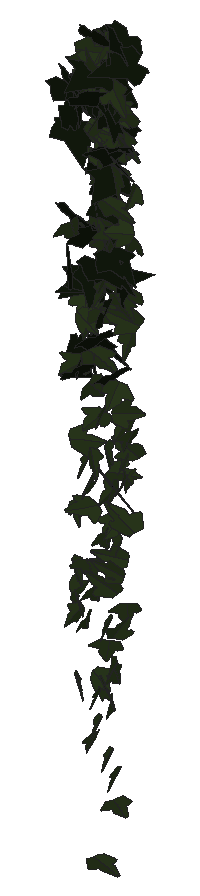
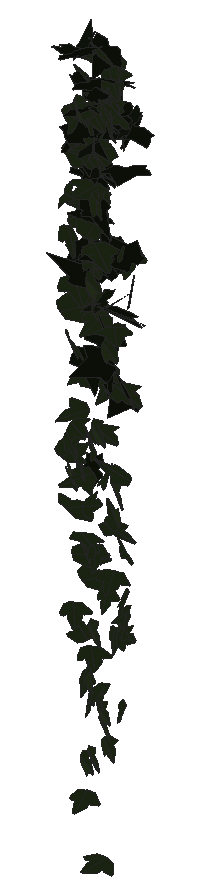
# SketchUp Ruby script. Lengths in inches.
U = 1.inch
M = Sketchup.active_model
def pt(a) = Geom::Point3d.new(a.map { |v| v * U })
def face(e, loops, mat)
  f = e.add_face(loops[0].map { |a| pt(a) })
  loops[1..].each { |l| e.add_face(l.map { |a| pt(a) }).erase! }
  f.material = f.back_material = mat if mat
  f
end
# faces: each face lists its corners as indices into pts; further lists are holes
def faces(e, pts, list, mat = nil) = list.each { |f| face(e, (f[0].is_a?(Array) ? f : [f]).map { |l| l.map { |i| pts[i] } }, mat) }
# xy, xz, yz: faces in a plane at the given z, y or x. An outline is a flat list of corners, or four numbers for a rectangle; further outlines are holes
def ring(l) = l.size == 4 ? [[l[0], l[1]], [l[2], l[1]], [l[2], l[3]], [l[0], l[3]]] : l.each_slice(2).to_a
def flat(e, list, mat, &to3) = list.each { |f| face(e, (f[0].is_a?(Array) ? f : [f]).map { |l| ring(l).map { |u, v| to3.(u, v) } }, mat) }
def xy(e, z, list, mat = nil) = flat(e, list, mat) { |x, y| [x, y, z] }
def xz(e, y, list, mat = nil) = flat(e, list, mat) { |x, z| [x, y, z] }
def yz(e, x, list, mat = nil) = flat(e, list, mat) { |y, z| [x, y, z] }
def lines(e, pts, list) = list.each { |a, b| e.add_line(pt(pts[a]), pt(pts[b])) }
# prism: a flat outline (further loops are holes) pulled along v
def prism(e, loops, v, mat = nil)
  f = face(e, loops, mat); d = Geom::Vector3d.new(v.map { |x| x * U })
  f.pushpull(f.normal.samedirection?(d) ? d.length : -d.length)
end
def box(e, o, s, mat = nil) = prism(e, [[o, [o[0] + s[0], o[1], o[2]], [o[0] + s[0], o[1] + s[1], o[2]], [o[0], o[1] + s[1], o[2]]]], [0, 0, s[2]], mat)
def at(x, y, z, deg = 0) = Geom::Transformation.translation(pt([x, y, z])) * Geom::Transformation.rotation(ORIGIN, Z_AXIS, deg.degrees)
def axes(o, x, y, z) = Geom::Transformation.new([*x, 0, *y, 0, *z, 0, *pt(o).to_a, 1])
def part(name) = M.definitions.add(name)
# library, detail: a bought-in or finely detailed component or shape, given as its bounding box
def library(name, o, s) = part(name).tap { |d| box(d.entities, o, s) }
def detail(e, o, s) = box(e.add_group.entities, o, s)
def put(e, d, t, mat = nil) = e.add_instance(d, t).tap { |i| i.material = mat if mat }
def group(e, t, mat = nil) = e.add_group.tap { |g| g.transformation = t; g.material = mat if mat }.entities
root = M.entities
M.materials.add("1026 AP 7946 SUNNY SIDE UP").color = [254, 231, 186]
M.materials.add("efeu1").color = [18, 25, 13]
M.materials.add("efeu2").color = [43, 57, 29]
c1 = part("ivyleaf_10")
p = [[0,0.5,-0.03],[-0.0625,2.02,-0.43],[-0.19,2.01,-0.46],[-0.54,1.05,-0.29],[-0.52,0.625,-0.18],[-0.83,0.76,-0.28],
  [-1.16,0.64,-0.33],[-1.15,0.33,-0.24],[-0.77,-0.39,0.02],[-0.3,-0.51,0.16],[0.04,-0.48,0.23],[-0.02,2.01,-0.4375],
  [-0.06,2.01,-0.43],[0.04,-0.49,0.23],[0.67,-0.49,0.14],[1.38,0.36,-0.2],[1.375,0.51,-0.24],[0.81,0.65,-0.19],
  [0.62,0.59,-0.15],[0.6,1.09,-0.28],[0.5,1.23,-0.31]]
faces(c1.entities,p,[[0,1,2,3,4,5,6,7,8,9,10],[11,12,0,13,14,15,16,17,18,19,20]],"efeu2")
c2 = part("ivyleaf_9")
p = [[1.54,2.16,1.25],[1.36,2.04,1.19],[-0.21,0.99,0.68],[-0.71,1.11,0.82],[-0.85,0.86,0.67],[-0.8,0.17,0.21],
  [-0.9,-0.01,0.1],[-0.67,-0.16,-0.02],[-0.08,-0.08,-0.05],[-0.03,-0.6,-0.4],[0.65,-0.88,-0.66],[0.83,-0.6,-0.49],
  [1.29,-0.42,-0.43],[1.8125,-0.07,-0.26],[1.21,0.44,0.15]]
faces(c2.entities,p,[[0,1,2,3,4,5,6,7,8,9,10,11,12,13,14]],"efeu1")
put(root,c1,axes([98.62,212.23,263.32],[-0.05399,0.08645,0.22814],[-0.03288,-0.21426,0.08745],[0.38721,-0.00614,0.03923]),"1026 AP 7946 SUNNY SIDE UP")
put(root,c2,axes([98,211.99,260.79],[0.05142,0.24508,-0.03116],[-0.00161,-0.03243,-0.26481],[-0.41963,0.03016,-0.0028]),"1026 AP 7946 SUNNY SIDE UP")
put(root,c1,axes([98.45,212.15,259.72],[0.16879,0.18196,-0.11803],[-0.09954,-0.09627,-0.22328],[-0.34936,0.11534,0.00659]),"1026 AP 7946 SUNNY SIDE UP")
put(root,c2,axes([98.13,212.12,257.58],[0.3163,-0.15076,0.02596],[0.01253,-0.03266,-0.25823],[0.24024,0.20019,-0.02071]),"1026 AP 7946 SUNNY SIDE UP")
put(root,c2,axes([97.9,212.27,266.85],[-0.38265,-0.11485,0.06292],[-0.02358,-0.09878,-0.25851],[0.21891,-0.21139,0.08214]),"1026 AP 7946 SUNNY SIDE UP")
put(root,c1,axes([98.48,212.1,255.43],[-0.08172,0.01136,-0.21221],[-0.32167,0.0251,0.05473],[0.04267,0.21102,0.00617]),"1026 AP 7946 SUNNY SIDE UP")
put(root,c2,axes([97.66,211.95,266.27],[0.24436,0.15063,0.08953],[0.11877,0.04568,-0.22161],[-0.2655,0.15907,-0.01674]),"1026 AP 7946 SUNNY SIDE UP")
put(root,c1,axes([98.14,212.25,258.12],[-0.02963,-0.00183,-0.24696],[0.14153,-0.22291,-0.00684],[-0.34936,-0.09015,0.01818]),"1026 AP 7946 SUNNY SIDE UP")
put(root,c1,axes([98.31,212.14,254.99],[-0.19456,-0.027,-0.19945],[-0.3045,-0.01293,0.12939],[-0.04009,0.22927,-0.01483]),"1026 AP 7946 SUNNY SIDE UP")
put(root,c2,axes([97.34,212.02,261.84],[-0.01147,-0.1083,0.21727],[0.07431,0.20015,0.1179],[-0.38551,0.0418,0.01626]),"1026 AP 7946 SUNNY SIDE UP")
put(root,c2,axes([97.97,212.1,262.51],[-0.02766,-0.0719,-0.2556],[0.30691,0.16003,-0.06283],[0.28926,-0.17667,0.04222]),"1026 AP 7946 SUNNY SIDE UP")
put(root,c1,axes([97.88,212.02,259.65],[-0.07653,-0.17148,-0.17777],[0.11044,0.15141,-0.18673],[0.38712,-0.07709,0.01813]),"1026 AP 7946 SUNNY SIDE UP")
put(root,c2,axes([98.41,212.01,260.07],[0.03333,0.24354,-0.01142],[0.00922,-0.01432,-0.26168],[-0.41399,0.01929,-0.00675]),"1026 AP 7946 SUNNY SIDE UP")
put(root,c1,axes([98.25,212.2,266.58],[0.27323,-0.01937,0.21405],[0.31451,-0.06212,-0.17856],[0.09415,0.26373,-0.0247]),"1026 AP 7946 SUNNY SIDE UP")
put(root,c1,axes([98.38,212.22,250.75],[0.08751,-0.17588,0.10202],[0.04332,-0.09619,-0.19059],[0.31519,0.06205,-0.00213]),"1026 AP 7946 SUNNY SIDE UP")
put(root,c2,axes([97.34,212.01,265.57],[-0.1105,-0.10868,0.24474],[0.15475,0.2117,0.13766],[-0.40318,0.11104,-0.01424]),"1026 AP 7946 SUNNY SIDE UP")
put(root,c1,axes([97.93,212.19,251.78],[0.13699,-0.1868,0.01947],[0.00085,-0.02175,-0.21228],[0.2954,0.08669,-0.00842]),"1026 AP 7946 SUNNY SIDE UP")
put(root,c2,axes([97.94,212.19,261.17],[-0.00846,0.16808,0.20737],[0.00268,-0.20036,0.17204],[0.41119,0.00476,0.00314]),"1026 AP 7946 SUNNY SIDE UP")
put(root,c2,axes([98.35,212.27,261.87],[0.01767,0.00567,0.23905],[0.06495,-0.2202,0.00101],[0.37343,0.03803,-0.01149]),"1026 AP 7946 SUNNY SIDE UP")
put(root,c1,axes([98.42,212.1,257.35],[0.09699,-0.19969,-0.10852],[-0.06043,0.09712,-0.21461],[0.34898,0.07232,-0.00701]),"1026 AP 7946 SUNNY SIDE UP")
put(root,c2,axes([97.61,212.03,266.04],[0.03478,-0.03634,-0.25666],[-0.36015,0.11283,-0.03622],[0.19765,0.21199,-0.02084]),"1026 AP 7946 SUNNY SIDE UP")
put(root,c1,axes([98.38,212.17,264.69],[-0.24639,0.18317,-0.05787],[-0.00052,-0.07102,-0.2469],[-0.32537,-0.13859,0.04421]),"1026 AP 7946 SUNNY SIDE UP")
put(root,c2,axes([98.14,212.35,265.875],[0.02863,-0.2037,0.17951],[0.01597,-0.17516,-0.21166],[0.42238,0.02043,-0.00416]),"1026 AP 7946 SUNNY SIDE UP")
put(root,c2,axes([98.34,212.12,262.79],[-0.01347,-0.15155,-0.18955],[0.02325,0.17457,-0.16],[0.39239,-0.01555,0.00297]),"1026 AP 7946 SUNNY SIDE UP")
put(root,c2,axes([98.29,212.28,264.54],[-0.36159,-0.10606,-0.02537],[0.05666,-0.01738,-0.25291],[0.17503,-0.21347,0.02947]),"1026 AP 7946 SUNNY SIDE UP")
put(root,c1,axes([98.21,212.27,263.17],[-0.18759,-0.14433,-0.1295],[-0.14599,-0.08364,0.19281],[-0.28209,0.13927,-0.01367]),"1026 AP 7946 SUNNY SIDE UP")
put(root,c1,axes([97.78,212.24,251.37],[0.01324,-0.20205,0.03394],[0,-0.03412,-0.20852],[0.32219,0.0083,-0.00139]),"1026 AP 7946 SUNNY SIDE UP")
put(root,c1,axes([97.67,212.34,263.52],[0.07905,-0.05436,0.2522],[0.30084,-0.15358,-0.07641],[0.25564,0.19755,0.01194]),"1026 AP 7946 SUNNY SIDE UP")
put(root,c2,axes([98.18,212.2,265.03],[0.05636,0.16822,-0.1752],[-0.07702,-0.15981,-0.1855],[-0.39353,0.05537,0.01121]),"1026 AP 7946 SUNNY SIDE UP")
put(root,c2,axes([98.76,212.32,267.28],[-0.41119,-0.03494,0.09096],[-0.13137,-0.05382,-0.25926],[0.08536,-0.25114,0.03918]),"1026 AP 7946 SUNNY SIDE UP")
put(root,c1,axes([98.46,212.22,261.75],[-0.28036,0.04766,-0.10327],[0.14484,-0.05147,-0.18317],[-0.11281,-0.18453,0.02147]),"1026 AP 7946 SUNNY SIDE UP")
put(root,c1,axes([97.28,212.36,254.0625],[-0.02084,-0.10696,0.18832],[0.04557,-0.18296,-0.10883],[0.33072,0.01847,0.02686]),"1026 AP 7946 SUNNY SIDE UP")
put(root,c1,axes([97.72,212.14,267.1],[-0.27462,0.11766,0.14744],[-0.22245,0.04851,-0.21084],[-0.20941,-0.20583,0.03061]),"1026 AP 7946 SUNNY SIDE UP")
put(root,c1,axes([97.84,212.16,254.83],[-0.07986,-0.18503,-0.09682],[0.0401,0.08937,-0.19714],[0.3231,-0.05682,0.00054]),"1026 AP 7946 SUNNY SIDE UP")
put(root,c1,axes([97.89,212.08,265.5625],[0.08814,-0.13085,0.215],[-0.09528,0.19492,0.15295],[-0.39808,-0.07562,0.01099]),"1026 AP 7946 SUNNY SIDE UP")
put(root,c1,axes([98.16,212.24,263.84],[-0.17266,-0.00024,-0.19243],[0.29858,-0.04267,-0.10709],[-0.06284,-0.20207,0.01989]),"1026 AP 7946 SUNNY SIDE UP")
put(root,c1,axes([97.57,212.125,261.07],[0.01749,0.18966,0.1305],[0.02246,0.11883,-0.2016],[-0.37981,0.01576,-0.00591]),"1026 AP 7946 SUNNY SIDE UP")
put(root,c1,axes([98.6875,212.34,261.23],[-0.13872,-0.07042,-0.24396],[-0.34189,-0.09637,0.1126],[-0.18317,0.2332,-0.02541]),"1026 AP 7946 SUNNY SIDE UP")
put(root,c1,axes([98.59,212.17,257.6],[0.05006,-0.16805,-0.13722],[-0.04213,0.12354,-0.18092],[0.35404,0.03846,-0.00213]),"1026 AP 7946 SUNNY SIDE UP")
put(root,c2,axes([98.22,212.45,267.5625],[0.20685,-0.15749,-0.16838],[0.1958,-0.10595,0.21053],[-0.32027,-0.16649,0.01996]),"1026 AP 7946 SUNNY SIDE UP")
put(root,c1,axes([97.6,212.17,267.23],[-0.06256,-0.00555,0.24261],[0.2995,0.14357,0.03647],[-0.2418,0.17926,-0.01759]),"1026 AP 7946 SUNNY SIDE UP")
put(root,c1,axes([97.93,212.21,248.54],[-0.21583,-0.07244,-0.13781],[0.20105,0.04167,-0.15865],[0.12856,-0.18679,0.01674]),"1026 AP 7946 SUNNY SIDE UP")
put(root,c1,axes([97.62,212.24,255.33],[-0.23729,-0.13098,-0.04733],[0.06898,0.01823,-0.20519],[0.20666,-0.15647,0.01415]),"1026 AP 7946 SUNNY SIDE UP")
put(root,c1,axes([98.68,212.25,256.54],[0.24744,0.07329,0.18747],[-0.28747,-0.02837,0.17488],[0.11019,-0.23858,0.03524]),"1026 AP 7946 SUNNY SIDE UP")
put(root,c1,axes([97.93,212.14,264.83],[0.05053,0.15207,-0.1553],[0.0059,0.14812,0.16682],[0.35905,-0.02383,0.01911]),"1026 AP 7946 SUNNY SIDE UP")
put(root,c1,axes([98.09,212.34,251.02],[0.14258,-0.17383,0.05277],[0.02323,-0.0511,-0.20201],[0.28445,0.09131,-0.00995]),"1026 AP 7946 SUNNY SIDE UP")
put(root,c1,axes([97.18,212.23,263.03],[-0.11836,-0.22763,-0.09502],[0.05265,0.08469,-0.24645],[0.38182,-0.08224,0.00453]),"1026 AP 7946 SUNNY SIDE UP")
put(root,c1,axes([97.93,212.36,267.57],[0.3567,-0.13818,0.05294],[0.04722,-0.05048,-0.27252],[0.22739,0.22723,-0.02646]),"1026 AP 7946 SUNNY SIDE UP")
put(root,c1,axes([97.34,212.37,259.83],[-0.20068,-0.09779,0.16638],[-0.15521,-0.13238,-0.16316],[0.25394,-0.15819,0.03176]),"1026 AP 7946 SUNNY SIDE UP")
put(root,c1,axes([98.37,212.37,255.63],[-0.02083,-0.03037,-0.21983],[-0.31453,-0.07743,0.02371],[-0.1255,0.1991,-0.02294]),"1026 AP 7946 SUNNY SIDE UP")
put(root,c1,axes([98.23,212.21,252.28],[0.0644,-0.14979,-0.13571],[0.01589,0.13502,-0.15514],[0.31236,0.02401,0.03587]),"1026 AP 7946 SUNNY SIDE UP")
put(root,c2,axes([98.09,212.18,265.98],[-0.07705,0.01589,-0.24506],[-0.38028,0.04839,0.05178],[0.08589,0.2285,0.00942]),"1026 AP 7946 SUNNY SIDE UP")
put(root,c1,axes([97.75,212.24,266.36],[0.38815,0.04154,-0.03196],[0.0427,0.03055,0.24774],[0.07622,-0.22863,0.02394]),"1026 AP 7946 SUNNY SIDE UP")
put(root,c2,axes([98.14,212.37,263.65],[-0.2159,-0.15152,-0.09996],[0.11916,0.06012,-0.21044],[0.27574,-0.14462,0.01267]),"1026 AP 7946 SUNNY SIDE UP")
put(root,c1,axes([97.58,212.23,254.02],[-0.01027,-0.17749,-0.11346],[-0.00497,0.10925,-0.18223],[0.32758,-0.0039,-0.00632]),"1026 AP 7946 SUNNY SIDE UP")
put(root,c1,axes([97.375,212.29,254.13],[-0.21574,0.1467,-0.03087],[-0.02042,0.02996,0.2068],[0.23481,0.13739,-0.01037]),"1026 AP 7946 SUNNY SIDE UP")
put(root,c2,axes([98.25,212.23,265.15],[0.17216,0.20859,-0.08239],[-0.10591,-0.05756,-0.24713],[-0.36395,0.11542,0.03294]),"1026 AP 7946 SUNNY SIDE UP")
put(root,c1,axes([97.76,212.29,260.2],[-0.23821,-0.07604,-0.16344],[0.25163,0.02607,-0.17061],[0.11344,-0.21749,0.03525]),"1026 AP 7946 SUNNY SIDE UP")
put(root,c2,axes([97.3,212.17,259.6875],[0.1768,0.18204,0.08713],[0.08414,0.06254,-0.22333],[-0.32619,0.1148,-0.01038]),"1026 AP 7946 SUNNY SIDE UP")
put(root,c2,axes([97.51,212.48,261.78],[-0.05418,-0.20603,0.08169],[-0.00563,-0.07936,-0.22414],[0.37453,-0.031,0.00845]),"1026 AP 7946 SUNNY SIDE UP")
put(root,c1,axes([97.8,212.43,258.73],[-0.17281,-0.10815,0.14958],[-0.07969,-0.14539,-0.1513],[0.2741,-0.11045,0.05031]),"1026 AP 7946 SUNNY SIDE UP")
put(root,c2,axes([97.72,212.27,267.63],[0.37484,0.00318,-0.1031],[-0.16164,-0.03026,-0.23514],[-0.02546,0.23901,-0.02501]),"1026 AP 7946 SUNNY SIDE UP")
put(root,c1,axes([97.55,212.37,267.11],[-0.10087,-0.25788,0.03069],[-0.00146,-0.03197,-0.27386],[0.40845,-0.0638,0.0066]),"1026 AP 7946 SUNNY SIDE UP")
put(root,c1,axes([98.31,212.29,249.98],[-0.18215,-0.14669,-0.08774],[0.10957,0.05178,-0.19108],[0.24245,-0.13361,0.02044]),"1026 AP 7946 SUNNY SIDE UP")
put(root,c1,axes([98.54,212.35,261.91],[-0.34665,-0.057,0.07993],[-0.10499,-0.05026,-0.2328],[0.10963,-0.22836,0.0298]),"1026 AP 7946 SUNNY SIDE UP")
put(root,c2,axes([97.63,212.16,266.08],[-0.1173,0.20286,-0.10074],[-0.04145,0.09384,0.23064],[0.37926,0.073,-0.00595]),"1026 AP 7946 SUNNY SIDE UP")
put(root,c1,axes([97.85,212.48,261.71],[0.02748,-0.15985,0.16939],[0.06568,-0.16085,-0.1657],[0.3556,0.04206,0.01751]),"1026 AP 7946 SUNNY SIDE UP")
put(root,c2,axes([97.87,212.44,264.89],[0.20256,-0.16122,0.16095],[0.14735,-0.12623,-0.21329],[0.32189,0.15924,-0.00365]),"1026 AP 7946 SUNNY SIDE UP")
put(root,c1,axes([98.03,212.4,254.03],[0.11701,-0.19939,0.03878],[0.01078,-0.03881,-0.21935],[0.3192,0.0744,-0.00681]),"1026 AP 7946 SUNNY SIDE UP")
put(root,c1,axes([97.79,212.44,252.45],[0.00736,-0.02061,0.21426],[0.29057,-0.09701,-0.01475],[0.15389,0.18416,0.0176]),"1026 AP 7946 SUNNY SIDE UP")
put(root,c1,axes([97.58,212.38,256.5625],[0.20694,-0.01456,-0.17655],[-0.27029,-0.0081,-0.13539],[0.00382,0.21586,-0.01572]),"1026 AP 7946 SUNNY SIDE UP")
put(root,c1,axes([98,212.49,262.15],[0.1061,-0.19436,0.14325],[0.04929,-0.13719,-0.21235],[0.37354,0.07331,-0.01267]),"1026 AP 7946 SUNNY SIDE UP")
put(root,c2,axes([98.15,212.32,262.1],[0.01533,0.02519,0.25238],[0.38209,-0.07398,-0.0018],[0.12465,0.22367,-0.02552]),"1026 AP 7946 SUNNY SIDE UP")
put(root,c2,axes([97.53,212.15,262.96],[-0.00897,0.11592,-0.24159],[-0.00378,0.23519,0.12087],[0.41225,0.00468,-0.00415]),"1026 AP 7946 SUNNY SIDE UP")
put(root,c1,axes([98.06,212.32,262.61],[-0.23805,0.15896,-0.0572],[-0.04292,0.05153,0.22711],[0.28257,0.14174,-0.01369]),"1026 AP 7946 SUNNY SIDE UP")
put(root,c1,axes([97.64,212.37,257.78],[-0.04609,0.22849,-0.0461],[0.00402,-0.0461,-0.23756],[-0.36648,-0.02924,0.0032]),"1026 AP 7946 SUNNY SIDE UP")
put(root,c2,axes([97.5,212.52,259.87],[-0.0261,0.01646,0.24858],[0.00772,-0.2417,0.01593],[0.38007,0.00604,0.01675]),"1026 AP 7946 SUNNY SIDE UP")
put(root,c1,axes([97.91,212.3,261.27],[-0.17229,-0.15629,-0.16254],[0.18441,0.10752,-0.1941],[0.29537,-0.1583,0.02638]),"1026 AP 7946 SUNNY SIDE UP")
put(root,c2,axes([96.97,212.5,263.01],[0.04354,-0.10361,0.2305],[0.23321,-0.17358,-0.10247],[0.31078,0.14478,0.0446]),"1026 AP 7946 SUNNY SIDE UP")
put(root,c1,axes([97.9,212.56,265.92],[-0.01434,0.01222,0.25091],[0.14817,-0.21736,0.01247],[0.36951,0.08763,0.00473]),"1026 AP 7946 SUNNY SIDE UP")
put(root,c1,axes([97.68,212.56,264.14],[0.03145,-0.13782,0.22095],[0.16394,-0.19274,-0.13823],[0.36695,0.09792,0.04282]),"1026 AP 7946 SUNNY SIDE UP")
put(root,c1,axes([97.24,212.39,252.43],[-0.1436,0.17685,-0.03693],[0.01337,-0.03704,-0.20504],[-0.28374,-0.09125,0.00903]),"1026 AP 7946 SUNNY SIDE UP")
put(root,c1,axes([97.26,212.23,254.57],[0.03256,-0.01377,-0.22601],[0.08042,0.21453,-0.00765],[0.33603,-0.05001,0.02373]),"1026 AP 7946 SUNNY SIDE UP")
put(root,c2,axes([96.93,212.53,266.23],[0.15041,-0.22236,0.10482],[0.04237,-0.10036,-0.24956],[0.383,0.09843,-0.01355]),"1026 AP 7946 SUNNY SIDE UP")
put(root,c1,axes([98.02,212.42,253.5],[-0.23098,-0.14832,0.01592],[-0.00047,-0.02257,-0.21458],[0.23461,-0.14606,0.01524]),"1026 AP 7946 SUNNY SIDE UP")
put(root,c1,axes([98.13,212.44,265.09],[0.36968,-0.11063,-0.02148],[-0.03834,-0.0034,-0.26117],[0.18655,0.21854,-0.01111]),"1026 AP 7946 SUNNY SIDE UP")
put(root,c1,axes([98.03,212.56,252.9375],[0.02295,-0.00625,0.21119],[0.15623,-0.17962,-0.01398],[0.28219,0.09995,-0.00944]),"1026 AP 7946 SUNNY SIDE UP")
put(root,c1,axes([97.39,212.4375,257.52],[0.12934,-0.18812,-0.00508],[-0.01127,0.00108,-0.21142],[0.29565,0.08234,-0.00583]),"1026 AP 7946 SUNNY SIDE UP")
put(root,c1,axes([98.32,212.53,265.29],[-0.10351,0.11551,0.1898],[0.13127,-0.15789,0.13759],[0.33205,0.09843,0.00477]),"1026 AP 7946 SUNNY SIDE UP")
put(root,c2,axes([97.46,212.51,261.76],[-0.37139,-0.04295,0.01087],[-0.00955,-0.0266,-0.23756],[0.07454,-0.21742,0.02371]),"1026 AP 7946 SUNNY SIDE UP")
put(root,c2,axes([97.08,212.5,265.14],[-0.14233,-0.22135,-0.10302],[0.08006,0.08569,-0.24546],[0.3726,-0.10296,0.01339]),"1026 AP 7946 SUNNY SIDE UP")
put(root,c1,axes([97.58,212.42,266.35],[-0.0182,-0.26249,-0.03601],[0.01773,0.03298,-0.2703],[0.4157,-0.0129,0.00995]),"1026 AP 7946 SUNNY SIDE UP")
put(root,c1,axes([97.7,212.51,252.28],[0.10415,-0.17627,0.08024],[0.02465,-0.07821,-0.19406],[0.30266,0.06703,-0.0118]),"1026 AP 7946 SUNNY SIDE UP")
put(root,c1,axes([98.24,212.44,255.95],[0.16812,-0.17744,-0.04009],[-0.04158,0.02829,-0.21309],[0.28225,0.10985,-0.00752]),"1026 AP 7946 SUNNY SIDE UP")
put(root,c1,axes([97.97,212.6,256.98],[-0.01993,-0.06027,0.22572],[0.07604,-0.21548,-0.05936],[0.34967,0.04343,0.02577]),"1026 AP 7946 SUNNY SIDE UP")
put(root,c2,axes([98.31,212.33,266.48],[-0.02916,0.0373,0.25233],[-0.23866,0.18875,-0.04041],[-0.3263,-0.14139,0.007]),"1026 AP 7946 SUNNY SIDE UP")
put(root,c1,axes([97.54,212.54,260.83],[0.02269,-0.19528,0.11158],[0.02478,-0.10849,-0.20224],[0.3511,0.02027,0.00706]),"1026 AP 7946 SUNNY SIDE UP")
put(root,c2,axes([96.95,212.42,266.14],[-0.09686,-0.08436,-0.24774],[0.28367,0.15962,-0.10456],[0.28203,-0.18952,0.02009]),"1026 AP 7946 SUNNY SIDE UP")
put(root,c1,axes([98.26,212.5,265.1],[-0.25382,-0.06604,0.18547],[-0.23106,-0.1136,-0.17287],[0.21569,-0.19941,0.03307]),"1026 AP 7946 SUNNY SIDE UP")
put(root,c1,axes([97.19,212.38,255.07],[-0.11982,0.21877,0.0409],[-0.03104,0.03383,-0.23834],[-0.34789,-0.07837,0.00718]),"1026 AP 7946 SUNNY SIDE UP")
put(root,c1,axes([97.65,212.37,266.66],[0.11373,-0.21544,-0.14817],[-0.06609,0.1363,-0.2333],[0.40084,0.0836,0.00357]),"1026 AP 7946 SUNNY SIDE UP")
put(root,c1,axes([97.38,212.46,256.77],[0.07068,-0.23344,-0.01028],[0.01646,-0.00679,0.24469],[-0.36695,-0.04527,0.00899]),"1026 AP 7946 SUNNY SIDE UP")
put(root,c1,axes([98.24,212.41,253.8],[-0.10659,-0.18527,0.07735],[0.03371,0.07321,0.20361],[-0.31315,0.07094,-0.00441]),"1026 AP 7946 SUNNY SIDE UP")
put(root,c1,axes([98.51,212.44,265.97],[-0.2254,0.00705,0.17651],[-0.27798,-0.03087,-0.14028],[0.0334,-0.20935,0.02364]),"1026 AP 7946 SUNNY SIDE UP")
put(root,c1,axes([97.96,212.5,262.78],[-0.11404,-0.21656,0.05335],[-0.01115,-0.05348,-0.23537],[0.3504,-0.07218,0.00987]),"1026 AP 7946 SUNNY SIDE UP")
put(root,c1,axes([97.78,212.35,252.71],[0.02158,0.18341,0.10076],[0.01883,0.09611,-0.18886],[-0.32553,0.01772,-0.00425]),"1026 AP 7946 SUNNY SIDE UP")
put(root,c1,axes([98.38,212.58,257.42],[-0.02849,-0.07193,-0.19715],[0.12141,-0.17988,0.06121],[-0.29701,-0.06663,0.04393]),"1026 AP 7946 SUNNY SIDE UP")
put(root,c2,axes([97.57,212.56,261.71],[-0.37222,0.00747,0.04452],[-0.0704,-0.07753,-0.22081],[0.0128,-0.20926,0.08007]),"1026 AP 7946 SUNNY SIDE UP")
put(root,c1,axes([98.35,212.57,258.71],[-0.07242,-0.1604,0.13979],[0.02955,-0.1424,-0.16656],[0.32996,-0.02245,0.0456]),"1026 AP 7946 SUNNY SIDE UP")
put(root,c1,axes([97.76,212.61,265.25],[0.15536,-0.09889,0.20944],[0.22242,-0.14682,-0.14485],[0.27832,0.17253,-0.00115]),"1026 AP 7946 SUNNY SIDE UP")
put(root,c1,axes([97.34,212.5,261.26],[0.25561,0.15073,-0.02551],[-0.01329,-0.02847,-0.22802],[-0.24003,0.16209,-0.01454]),"1026 AP 7946 SUNNY SIDE UP")
put(root,c1,axes([97.79,212.57,264.2],[0.00668,-0.24233,0.08681],[0.02099,-0.08533,-0.24992],[0.4036,0.00845,0.01156]),"1026 AP 7946 SUNNY SIDE UP")
put(root,c1,axes([98.33,212.52,257.89],[0.18339,-0.17034,0.01561],[-0.00107,-0.01997,-0.21244],[0.26903,0.11603,-0.01148]),"1026 AP 7946 SUNNY SIDE UP")
put(root,c1,axes([97.81,212.56,258.84],[0.10625,-0.2018,0.06857],[0.01922,-0.06724,-0.21942],[0.33414,0.06804,-0.00918]),"1026 AP 7946 SUNNY SIDE UP")
put(root,c1,axes([98.23,212.52,265.32],[-0.25955,0.08482,-0.17471],[0.22496,-0.0984,-0.18779],[-0.21889,-0.20171,0.01416]),"1026 AP 7946 SUNNY SIDE UP")
put(root,c2,axes([97.08,212.59,260.125],[-0.18932,-0.00177,-0.22167],[0.3275,-0.06288,-0.1199],[-0.08496,-0.23841,0.03178]),"1026 AP 7946 SUNNY SIDE UP")
put(root,c1,axes([97.15,212.5,257.92],[0.11195,-0.05817,-0.22439],[0.34193,-0.04128,0.08447],[-0.09164,-0.22509,0.04105]),"1026 AP 7946 SUNNY SIDE UP")
put(root,c1,axes([97.9,212.51,264.42],[-0.31181,-0.07831,-0.14641],[0.25896,-0.04149,-0.19596],[0.06088,-0.2246,0.08363]),"1026 AP 7946 SUNNY SIDE UP")
put(root,c1,axes([98.15,212.44,252.89],[-0.01638,-0.1812,-0.0983],[0.05245,0.09173,-0.18468],[0.31695,-0.02455,0.02548]),"1026 AP 7946 SUNNY SIDE UP")
put(root,c1,axes([97.78,212.56,263.04],[-0.27276,-0.15656,0.09495],[-0.07298,-0.08627,-0.23916],[0.27693,-0.17694,0.0305]),"1026 AP 7946 SUNNY SIDE UP")
put(root,c2,axes([97.89,212.61,265.48],[0.18158,-0.18272,0.1252],[0.09467,-0.10689,-0.22324],[0.33276,0.13012,-0.00481]),"1026 AP 7946 SUNNY SIDE UP")
put(root,c1,axes([98.24,212.59,266.25],[0.12699,-0.23215,0.05819],[0.02416,-0.05585,-0.25352],[0.3754,0.08213,-0.00337]),"1026 AP 7946 SUNNY SIDE UP")
put(root,c1,axes([98.63,212.45,263.1],[-0.26837,0.10757,0.13273],[-0.20114,0.04154,-0.20206],[-0.19022,-0.19569,0.02639]),"1026 AP 7946 SUNNY SIDE UP")
put(root,c1,axes([98.08,212.4,265.95],[0.14733,0.16645,0.17426],[0.12092,0.14396,-0.19894],[-0.37355,0.11225,0.00433]),"1026 AP 7946 SUNNY SIDE UP")
put(root,c1,axes([98.54,212.63,264.1],[0.03148,0.12924,-0.17372],[-0.0619,-0.16006,-0.14173],[-0.34894,0.04005,0.00947]),"1026 AP 7946 SUNNY SIDE UP")
put(root,c2,axes([97.875,212.67,266.9375],[-0.22535,-0.20045,0.03194],[-0.01564,-0.03279,-0.25761],[0.34434,-0.13267,0.00921]),"1026 AP 7946 SUNNY SIDE UP")
put(root,c1,axes([98,212.47,263.01],[0.10183,-0.21583,-0.11911],[-0.0344,0.11275,-0.23124],[0.38255,0.06759,0.01091]),"1026 AP 7946 SUNNY SIDE UP")
put(root,c1,axes([97.67,212.47,265.39],[-0.13484,-0.0798,-0.24535],[0.37768,0.04595,-0.10489],[0.11314,-0.24849,0.05774]),"1026 AP 7946 SUNNY SIDE UP")
put(root,c2,axes([98.0625,212.65,266.25],[-0.16392,-0.22708,-0.02198],[0.02098,0.01593,-0.25726],[0.35784,-0.10495,0.00501]),"1026 AP 7946 SUNNY SIDE UP")
put(root,c1,axes([98.41,212.53,254.44],[-0.19544,-0.16606,-0.00721],[0.01838,-0.00119,-0.21344],[0.26064,-0.12443,0.00965]),"1026 AP 7946 SUNNY SIDE UP")
put(root,c2,axes([97.6,212.5,260.43],[0.38541,-0.04915,0.0329],[0.04194,-0.03009,-0.25652],[0.08233,0.24538,-0.02335]),"1026 AP 7946 SUNNY SIDE UP")
put(root,c1,axes([98.38,212.625,260.69],[0.27583,-0.14427,0.09735],[0.09063,-0.07922,-0.23328],[0.25634,0.18325,-0.02227]),"1026 AP 7946 SUNNY SIDE UP")
put(root,c2,axes([97.55,212.57,261.93],[0.21426,-0.18564,-0.02326],[-0.00508,0.02129,-0.23981],[0.31678,0.1259,0.01189]),"1026 AP 7946 SUNNY SIDE UP")
put(root,c2,axes([97.98,212.46,264.07],[0.12565,0.03827,-0.2554],[-0.3885,-0.03429,-0.08762],[-0.07016,0.25842,0.02777]),"1026 AP 7946 SUNNY SIDE UP")
put(root,c1,axes([97.85,212.5,255.96],[-0.05058,-0.2077,-0.07836],[0.04185,0.07147,-0.21558],[0.34463,-0.03916,0.01468]),"1026 AP 7946 SUNNY SIDE UP")
put(root,c1,axes([96.99,212.625,256.29],[0.19801,-0.07286,0.1464],[0.18622,-0.07957,-0.15018],[0.16931,0.17273,-0.00603]),"1026 AP 7946 SUNNY SIDE UP")
put(root,c1,axes([98.53,212.6,258.02],[-0.20622,-0.06147,-0.1636],[-0.24531,-0.03587,0.14715],[-0.10603,0.20254,-0.02226]),"1026 AP 7946 SUNNY SIDE UP")
put(root,c2,axes([98.24,212.73,267.54],[-0.21446,-0.20058,0.08462],[-0.03808,-0.08368,-0.24898],[0.33937,-0.13615,0.02554]),"1026 AP 7946 SUNNY SIDE UP")
put(root,c1,axes([98.16,212.42,257.55],[-0.08625,-0.07964,-0.23336],[0.2455,0.16409,-0.09762],[0.28596,-0.1649,0.01342]),"1026 AP 7946 SUNNY SIDE UP")
put(root,c2,axes([98.27,212.57,265.6875],[0.06807,0.03528,-0.2285],[-0.28914,-0.12943,-0.05885],[-0.22765,0.17494,0.00642]),"1026 AP 7946 SUNNY SIDE UP")
put(root,c1,axes([97.22,212.62,266.38],[0.30903,-0.01582,0.16761],[0.2562,-0.05132,-0.19388],[0.07684,0.2347,-0.02765]),"1026 AP 7946 SUNNY SIDE UP")
put(root,c1,axes([97.98,212.56,266.25],[-0.3017,-0.01497,0.13359],[-0.20727,-0.03205,-0.19044],[0.05192,-0.21489,0.01602]),"1026 AP 7946 SUNNY SIDE UP")
put(root,c1,axes([98.34,212.38,258.98],[0.02244,0.04616,0.25113],[0.05001,0.24155,-0.04768],[-0.38649,0.03394,0.00841]),"1026 AP 7946 SUNNY SIDE UP")
put(root,c1,axes([98.4375,212.61,258.43],[-0.03307,-0.2072,0.03323],[0.00292,-0.03378,-0.21468],[0.33,-0.02046,0.00523]),"1026 AP 7946 SUNNY SIDE UP")
put(root,c1,axes([98.05,212.61,256.26],[0.30736,0.03192,-0.07083],[-0.10187,-0.0293,-0.20342],[-0.06237,0.20519,-0.01677]),"1026 AP 7946 SUNNY SIDE UP")
